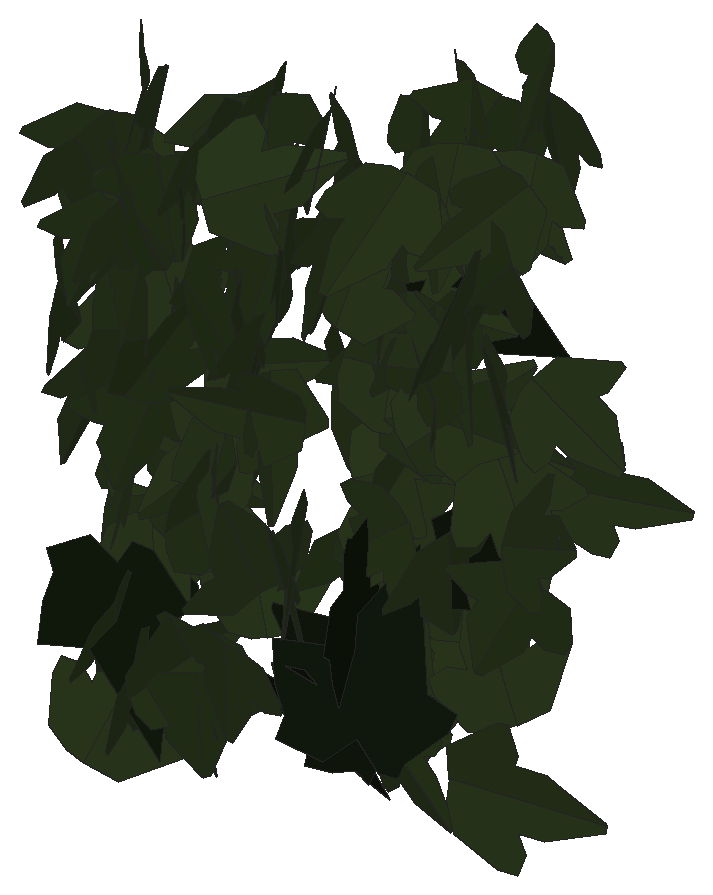
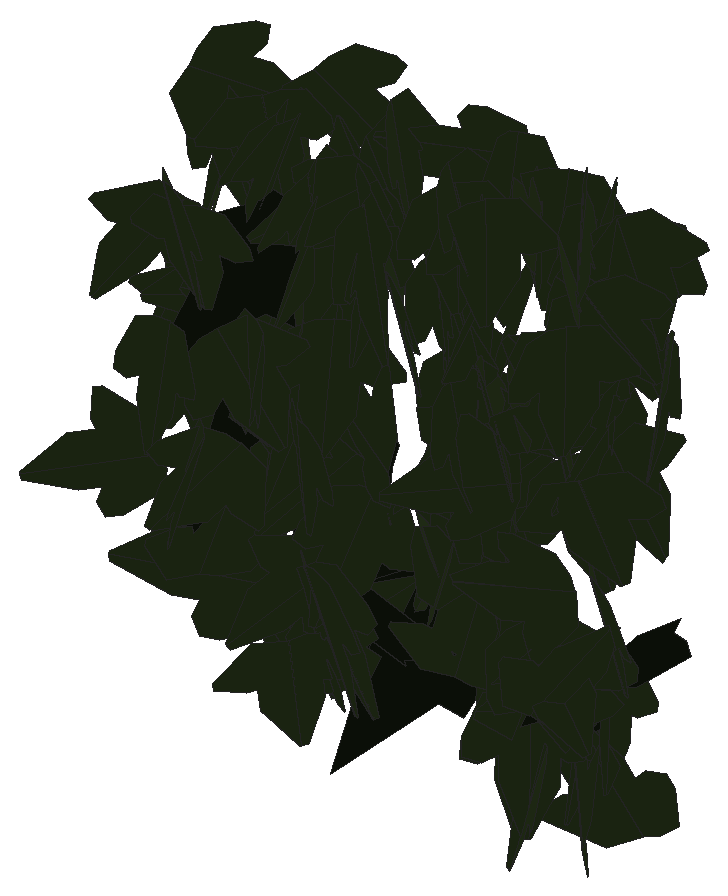
# SketchUp Ruby script. Lengths in inches.
U = 1.inch
M = Sketchup.active_model
def pt(a) = Geom::Point3d.new(a.map { |v| v * U })
def face(e, loops, mat)
  f = e.add_face(loops[0].map { |a| pt(a) })
  loops[1..].each { |l| e.add_face(l.map { |a| pt(a) }).erase! }
  f.material = f.back_material = mat if mat
  f
end
# faces: each face lists its corners as indices into pts; further lists are holes
def faces(e, pts, list, mat = nil) = list.each { |f| face(e, (f[0].is_a?(Array) ? f : [f]).map { |l| l.map { |i| pts[i] } }, mat) }
# xy, xz, yz: faces in a plane at the given z, y or x. An outline is a flat list of corners, or four numbers for a rectangle; further outlines are holes
def ring(l) = l.size == 4 ? [[l[0], l[1]], [l[2], l[1]], [l[2], l[3]], [l[0], l[3]]] : l.each_slice(2).to_a
def flat(e, list, mat, &to3) = list.each { |f| face(e, (f[0].is_a?(Array) ? f : [f]).map { |l| ring(l).map { |u, v| to3.(u, v) } }, mat) }
def xy(e, z, list, mat = nil) = flat(e, list, mat) { |x, y| [x, y, z] }
def xz(e, y, list, mat = nil) = flat(e, list, mat) { |x, z| [x, y, z] }
def yz(e, x, list, mat = nil) = flat(e, list, mat) { |y, z| [x, y, z] }
def lines(e, pts, list) = list.each { |a, b| e.add_line(pt(pts[a]), pt(pts[b])) }
# prism: a flat outline (further loops are holes) pulled along v
def prism(e, loops, v, mat = nil)
  f = face(e, loops, mat); d = Geom::Vector3d.new(v.map { |x| x * U })
  f.pushpull(f.normal.samedirection?(d) ? d.length : -d.length)
end
def box(e, o, s, mat = nil) = prism(e, [[o, [o[0] + s[0], o[1], o[2]], [o[0] + s[0], o[1] + s[1], o[2]], [o[0], o[1] + s[1], o[2]]]], [0, 0, s[2]], mat)
def at(x, y, z, deg = 0) = Geom::Transformation.translation(pt([x, y, z])) * Geom::Transformation.rotation(ORIGIN, Z_AXIS, deg.degrees)
def axes(o, x, y, z) = Geom::Transformation.new([*x, 0, *y, 0, *z, 0, *pt(o).to_a, 1])
def part(name) = M.definitions.add(name)
# library, detail: a bought-in or finely detailed component or shape, given as its bounding box
def library(name, o, s) = part(name).tap { |d| box(d.entities, o, s) }
def detail(e, o, s) = box(e.add_group.entities, o, s)
def put(e, d, t, mat = nil) = e.add_instance(d, t).tap { |i| i.material = mat if mat }
def group(e, t, mat = nil) = e.add_group.tap { |g| g.transformation = t; g.material = mat if mat }.entities
root = M.entities
M.materials.add("efeu1").color = [18, 25, 13]
M.materials.add("efeu2").color = [43, 57, 29]
c1 = part("ivyleaf_10")
p = [[0,0.5,-0.03],[-0.0625,2.02,-0.43],[-0.19,2.01,-0.46],[-0.54,1.05,-0.29],[-0.52,0.625,-0.18],[-0.83,0.76,-0.28],
  [-1.16,0.64,-0.33],[-1.15,0.33,-0.24],[-0.77,-0.39,0.02],[-0.3,-0.51,0.16],[0.04,-0.48,0.23],[-0.02,2.01,-0.4375],
  [-0.06,2.01,-0.43],[0.04,-0.49,0.23],[0.67,-0.49,0.14],[1.38,0.36,-0.2],[1.375,0.51,-0.24],[0.81,0.65,-0.19],
  [0.62,0.59,-0.15],[0.6,1.09,-0.28],[0.5,1.23,-0.31]]
faces(c1.entities,p,[[0,1,2,3,4,5,6,7,8,9,10],[11,12,0,13,14,15,16,17,18,19,20]],"efeu2")
c2 = part("ivyleaf_9")
p = [[1.54,2.16,1.25],[1.36,2.04,1.19],[-0.21,0.99,0.68],[-0.71,1.11,0.82],[-0.85,0.86,0.67],[-0.8,0.17,0.21],
  [-0.9,-0.01,0.1],[-0.67,-0.16,-0.02],[-0.08,-0.08,-0.05],[-0.03,-0.6,-0.4],[0.65,-0.88,-0.66],[0.83,-0.6,-0.49],
  [1.29,-0.42,-0.43],[1.8125,-0.07,-0.26],[1.21,0.44,0.15]]
faces(c2.entities,p,[[0,1,2,3,4,5,6,7,8,9,10,11,12,13,14]],"efeu1")
put(root,c1,axes([517.64,137.4375,171.26],[-0.41688,-0.46521,0.2029],[-0.12447,-0.16084,-0.62452],[0.49204,-0.43484,0.01392]))
put(root,c1,axes([517.58,138.02,170.76],[0.50055,0.26687,-0.30251],[-0.27279,-0.13124,-0.56713],[-0.29719,0.56995,0.01106]))
put(root,c1,axes([517.57,136.68,169.37],[0.25676,-0.43077,-0.48205],[-0.05354,0.50272,-0.47777],[0.64426,0.21346,0.15241]))
put(root,c1,axes([517.52,138.27,168.3],[0.55314,0.38276,-0.16418],[-0.12927,-0.1017,-0.67259],[-0.39592,0.56796,-0.00978]))
put(root,c1,axes([517.625,137.09,171.14],[-0.27738,-0.54194,-0.30528],[0.1181,0.2823,-0.60844],[0.6107,-0.30074,-0.021]))
put(root,c1,axes([517.77,137.28,168.16],[0.02051,-0.62852,0.23191],[0.01492,-0.23153,-0.62881],[0.66977,0.02441,0.0069]))
put(root,c1,axes([517.74,138.43,170.21],[-0.36359,-0.52843,0.00032],[0.09695,-0.06709,-0.6305],[0.51946,-0.35734,0.1179]))
put(root,c1,axes([517.9375,137.78,171.82],[0.11467,-0.29115,-0.5829],[-0.19247,0.55031,-0.31273],[0.62249,0.22379,0.01068]))
put(root,c1,axes([517.8125,137.65,166.57],[0.49001,-0.44367,0.04357],[0.03635,-0.02476,-0.661],[0.44432,0.49132,0.00603]))
put(root,c1,axes([518.02,137.22,170.3],[-0.24186,-0.56119,0.25106],[-0.10207,-0.22939,-0.61109],[0.60626,-0.2625,-0.00272]))
put(root,c1,axes([517.92,137.14,168.78],[0.08283,-0.33916,-0.69143],[0.11937,0.69267,-0.32546],[0.76083,-0.07175,0.12634]))
put(root,c1,axes([517.83,138.25,171.48],[0.29503,-0.48495,0.30679],[0.20898,-0.23047,-0.56529],[0.53443,0.35784,0.05169]))
put(root,c1,axes([517.69,138.11,163.74],[-0.17301,0.10333,0.67463],[0.5676,-0.36467,0.20141],[0.37898,0.59335,0.00631]))
put(root,c1,axes([518.25,138.12,165.25],[0.33526,0.43245,0.34069],[-0.20578,-0.27154,0.54718],[0.51062,-0.39337,-0.00318]))
put(root,c1,axes([518.2,136.93,165.01],[0.05391,-0.58364,-0.27077],[-0.01616,0.2704,-0.58607],[0.64319,0.05571,0.00797]))
put(root,c1,axes([518.49,138.06,165.82],[-0.49926,-0.31226,0.34526],[-0.2853,-0.19481,-0.58875],[0.36786,-0.5749,0.01198]))
put(root,c1,axes([518.2,137.67,170.58],[-0.05586,-0.45061,0.49221],[0.07276,-0.4951,-0.445],[0.66335,0.01636,0.09026]))
put(root,c1,axes([518.41,137.38,167.77],[-0.42657,-0.46754,0.19759],[-0.13608,-0.1433,-0.63288],[0.489,-0.44773,-0.00377]))
put(root,c1,axes([518.29,137.99,168.83],[0.29373,0.60761,0.09095],[-0.04537,-0.07908,0.67485],[0.6127,-0.29715,0.00637]))
put(root,c1,axes([518.34,137.83,168.84],[0.36132,-0.5316,-0.13386],[-0.06634,0.11675,-0.64268],[0.54417,0.36721,0.01054]))
put(root,c1,axes([518.16,137.77,165.625],[0.44886,0.5418,-0.00013],[-0.0055,0.00439,-0.70355],[-0.54178,0.44884,0.00704]))
put(root,c1,axes([517.99,136.96,163.29],[0.65454,0.19171,-0.32038],[0.30766,0.08937,0.68204],[0.21152,-0.72324,-0.00064]))
put(root,c1,axes([518.32,137.14,169.51],[0.5315,-0.32105,-0.18696],[-0.08148,0.21767,-0.60539],[0.36248,0.51968,0.13806]))
put(root,c2,axes([518.04,137.26,165.41],[0.04679,-0.74995,-0.27279],[-0.01333,0.27249,-0.7514],[0.79791,0.04853,0.00345]))
put(root,c1,axes([518.4375,136.9,170.65],[-0.14155,-0.58604,-0.38884],[0.11696,0.3715,-0.60248],[0.69351,-0.18227,0.02224]))
put(root,c1,axes([518.61,136.95,170.3],[-0.45453,0.48299,-0.05741],[-0.05818,0.02403,0.66273],[0.4829,0.45751,0.0258]))
put(root,c1,axes([518.67,136.78,164.39],[0.11905,-0.52024,-0.41216],[0.00472,0.41939,-0.528],[0.6637,0.09034,0.07768]))
put(root,c1,axes([518.27,138.12,166.72],[-0.15942,0.0089,-0.64339],[0.63789,-0.08478,-0.15923],[-0.08442,-0.65741,0.01183]))
put(root,c1,axes([518.77,137.75,163.97],[-0.47433,0.45423,0.01807],[-0.01388,0.01164,-0.65674],[-0.45437,-0.47453,0.0012]))
put(root,c1,axes([518.71,138.03,169.38],[0.22855,-0.52585,0.28258],[0.13003,-0.25147,-0.57312],[0.58264,0.26239,0.01706]))
put(root,c1,axes([518.99,137.62,164.53],[-0.68946,-0.12038,0.12223],[-0.11902,-0.02894,-0.69985],[0.12355,-0.69961,0.00792]))
put(root,c1,axes([518.92,137.02,171.28],[-0.59463,-0.30584,-0.02832],[0.02471,0.01388,-0.66867],[0.30615,-0.59514,-0.00104]))
put(root,c1,axes([518.74,136.95,168.48],[-0.01587,-0.60564,0.37816],[0.0675,0.37529,0.60387],[-0.71081,0.04916,0.0489]))
put(root,c1,axes([518.98,138.34,169.26],[0.36772,-0.53312,-0.12379],[-0.07433,0.09911,-0.64762],[0.54223,0.37512,-0.00482]))
put(root,c1,axes([518.96,138.42,171.5],[-0.40198,-0.4968,0.02458],[0.08605,-0.10059,-0.62568],[0.48991,-0.38997,0.13007]))
put(root,c1,axes([518.95,136.87,164.32],[0.02781,-0.25459,0.6538],[0.00815,0.65438,0.25447],[-0.70157,-0.00249,0.02887]))
put(root,c1,axes([518.88,137.65,170.89],[0.0621,-0.27819,-0.60931],[0.17844,-0.58294,0.28433],[-0.64561,-0.18787,0.01998]))
put(root,c1,axes([519.21,137.68,167.23],[-0.15559,-0.09227,0.6372],[0.07092,-0.654,-0.07739],[0.63992,0.05005,0.1635]))
put(root,c1,axes([519.32,137.19,164.24],[-0.50827,-0.44501,-0.02178],[0.01647,0.01426,-0.67555],[0.44523,-0.50854,0.00012]))
put(root,c1,axes([519.12,141.61,169.97],[0.52221,-0.3603,0.08583],[0.12676,0.03446,-0.6266],[0.34802,0.52809,0.09944]))
put(root,c1,axes([518.94,138.34,168.02],[0.02994,-0.04889,0.63892],[0.309,0.56144,0.02849],[-0.56136,0.30643,0.04976]))
put(root,c1,axes([519.32,138.48,168.97],[0.02159,-0.63533,0.02516],[0.02441,-0.02433,-0.63526],[0.63536,0.02252,0.02355]))
put(root,c1,axes([519.36,137.3,171.73],[-0.02289,-0.62057,-0.32602],[0.0194,0.32551,-0.62095],[0.70072,-0.02928,0.00655]))
put(root,c1,axes([519.37,138.48,171.6],[-0.40551,-0.48926,0.03021],[0.04309,-0.07463,-0.63031],[0.48829,-0.39972,0.08071]))
put(root,c1,axes([519.36,138.43,171.88],[0.11507,-0.62928,0.02192],[0.00385,-0.02158,-0.63971],[0.62965,0.11514,-0.0001]))
put(root,c1,axes([519.55,137.73,169.84],[0.04002,-0.10856,-0.66867],[-0.0739,0.66514,-0.11241],[0.67338,0.07945,0.0274]))
put(root,c1,axes([519.14,137.74,167.3],[0.0355,-0.02653,-0.64087],[0.27993,-0.57686,0.03938],[-0.57711,-0.28144,-0.02031]))
put(root,c1,axes([519.54,136.96,169.83],[-0.3289,0.54085,0.3855],[-0.192,0.33438,-0.63295],[-0.63581,-0.38075,-0.00828]))
put(root,c1,axes([519.53,136.68,166.81],[0.02424,0.02111,0.65659],[-0.22978,0.6158,-0.01132],[-0.61543,-0.22909,0.03009]))
put(root,c1,axes([519.85,137.75,169.22],[0.23119,-0.09019,0.62127],[-0.58524,0.20861,0.24807],[-0.22717,-0.62921,-0.0068]))
put(root,c1,axes([519.42,138.15,167.35],[-0.06097,-0.02228,0.65518],[0.31749,-0.57669,0.00994],[0.57355,0.31686,0.06415]))
put(root,c1,axes([519.56,137.43,167.72],[0.25378,0.61188,-0.14748],[-0.05329,-0.13756,-0.66241],[-0.62714,0.25929,-0.00339]))
put(root,c1,axes([519.72,137.94,165.18],[0.57225,0.27682,0.15029],[-0.13842,-0.05897,0.63565],[0.28294,-0.58871,0.007]))
put(root,c1,axes([519.8,137.72,169.11],[0.09402,-0.6424,0.03786],[0.00407,-0.03767,-0.64925],[0.64351,0.0941,-0.00143]))
put(root,c1,axes([519.93,138.01,170.28],[-0.14502,-0.61082,0.15015],[-0.03017,-0.14715,-0.62778],[0.62827,-0.14805,0.00451]))
put(root,c1,axes([520.03,136.91,165.01],[-0.6357,0.03884,0.16465],[-0.16466,0.00483,-0.63686],[-0.03881,-0.65666,0.00505]))
put(root,c1,axes([520.33,137.43,168.22],[-0.13923,0.09197,-0.63195],[-0.62403,-0.15699,0.11463],[-0.13566,0.62777,0.12125]))
put(root,c1,axes([519.99,137.49,165.91],[-0.30786,-0.56385,-0.32507],[-0.14344,-0.29198,0.64229],[-0.63484,0.3394,0.01251]))
put(root,c1,axes([519.91,138.03,170.32],[0.39093,-0.51019,-0.0648],[0.05112,0.11954,-0.63278],[0.51174,0.3778,0.11272]))
put(root,c1,axes([519.92,141.5625,170.86],[-0.46716,0.41506,-0.1659],[0.04195,-0.1982,-0.614],[-0.44501,-0.4544,0.11628]))
put(root,c1,axes([519.9,137.94,168.07],[-0.02344,0.68269,-0.2239],[0.01447,-0.22352,-0.68306],[-0.71832,-0.02678,-0.00645]))
put(root,c1,axes([520.42,138.91,171.07],[-0.49785,0.20256,0.52864],[-0.50472,0.16004,-0.53665],[-0.25641,-0.70831,0.02992]))
put(root,c1,axes([520.33,141.51,170.66],[-0.41762,-0.37017,0.33114],[-0.21401,-0.2563,-0.55642],[0.44819,-0.4673,0.04287]))
put(root,c1,axes([520.34,137.52,170.77],[0.00828,0.21516,-0.621],[-0.17314,0.59982,0.20552],[0.634,0.161,0.06424]))
put(root,c1,axes([520.15,142.44,169.74],[-0.31556,0.55437,-0.02515],[0.02061,-0.01721,-0.63782],[-0.55455,-0.31609,-0.00939]))
put(root,c1,axes([520.29,138.41,170.125],[0.44141,-0.46826,-0.02029],[-0.00115,0.02678,-0.64328],[0.4687,0.44107,0.01752]))
put(root,c1,axes([520.14,141.92,169.46],[-0.45097,-0.22462,-0.39564],[0.41045,0.03946,-0.49025],[0.19627,-0.59863,0.11614]))
put(root,c1,axes([519.99,136.97,171.48],[0.19355,-0.00511,-0.67426],[0.58077,0.35766,0.164],[0.34258,-0.60346,0.10291]))
put(root,c1,axes([520.58,137.99,172.07],[0.20739,-0.62861,-0.08831],[-0.01157,0.08915,-0.66172],[0.63468,0.20703,0.01679]))
put(root,c1,axes([520.375,137.47,166.28],[-0.37386,0.46001,-0.27352],[0.18004,-0.2061,-0.5927],[-0.50399,-0.41486,-0.00884]))
put(root,c1,axes([520.65,138.36,170.49],[0.06241,-0.59673,-0.24058],[0.10624,0.24795,-0.58745],[0.63457,0.01718,0.12201]))
put(root,c1,axes([520.53,137.57,166.7],[0.28508,-0.28805,0.53632],[0.38759,-0.37081,-0.40517],[0.46946,0.48105,0.00883]))
put(root,c1,axes([520.33,138.65,168.07],[-0.10454,-0.0025,0.74605],[0.71745,-0.20696,0.09984],[0.20463,0.72435,0.0311]))
put(root,c1,axes([521.01,141.96,170.71],[-0.61169,0.19732,0.08542],[-0.08791,0.00557,-0.64237],[-0.19623,-0.6176,0.0215]))
put(root,c1,axes([521.15,138.71,165.92],[0.56927,-0.28984,-0.4175],[-0.35146,0.22834,-0.63774],[0.36713,0.66801,0.03685]))
put(root,c2,axes([520.75,137.01,164.91],[0.74936,0.1265,-0.10238],[-0.10095,-0.01703,-0.75996],[-0.12764,0.75613,0.00002]))
put(root,c1,axes([521.2,138.71,165.92],[0.5832,-0.47068,-0.14626],[-0.11538,0.08991,-0.74943],[0.47918,0.5945,-0.00245]))
put(root,c1,axes([521.14,137.99,166.63],[-0.37029,-0.48383,-0.30882],[0.18133,0.25008,-0.60922],[0.54459,-0.41224,-0.00713]))
put(root,c1,axes([521.32,138.375,169.02],[-0.46453,-0.45378,-0.04907],[0.02882,0.04071,-0.64933],[0.45552,-0.46534,-0.00896]))
put(root,c1,axes([521.29,137.49,171.17],[0.10146,-0.62963,0.21567],[0.07532,-0.20589,-0.63653],[0.66127,0.12006,0.03941]))
put(root,c2,axes([521.93,137.35,164.93],[-0.53326,-0.03605,-0.56706],[-0.55591,-0.12779,0.5309],[-0.11755,0.76784,0.06173]))
put(root,c1,axes([521.58,140.96,171.99],[0.45997,-0.43119,-0.08942],[-0.05346,0.07367,-0.63024],[0.43711,0.46275,0.01702]))
put(root,c1,axes([521.69,138.05,164.73],[0.02404,0.2892,0.67807],[-0.07076,-0.6744,0.29014],[0.73377,-0.07451,0.00577]))
put(root,c1,axes([521.32,137.98,170.93],[-0.1875,-0.20395,-0.57631],[0.48447,0.31807,-0.27018],[0.37285,-0.51586,0.06125]))
put(root,c1,axes([522.01,137.49,167.27],[0.39783,-0.14512,-0.48941],[-0.43301,0.23265,-0.42098],[0.27033,0.58623,0.04592]))
put(root,c1,axes([521.53,137.32,170.33],[0.66433,-0.11572,-0.11217],[0.1173,0.02094,0.67313],[-0.11051,-0.6734,0.0402]))
put(root,c1,axes([521.65,138.42,171.1],[0.00527,0.59662,-0.23108],[-0.0124,-0.23095,-0.59656],[-0.63969,0.0094,0.00966]))
put(root,c2,axes([521.93,136.76,166.6875],[0.12356,-0.06211,-0.76596],[-0.62775,0.43933,-0.13689],[0.44326,0.63949,0.01965]))
put(root,c1,axes([521.69,138.65,164.85],[0.44545,0.50513,-0.06677],[-0.04805,-0.04665,-0.67347],[-0.50726,0.448,0.00516]))
put(root,c1,axes([521.77,138.15,168.03],[-0.10534,-0.50237,-0.46448],[0.10769,0.45192,-0.51321],[0.67567,-0.15035,0.00938]))
put(root,c1,axes([521.78,137.95,170.375],[0.12684,-0.4773,-0.50678],[0.09194,0.52209,-0.46871],[0.69006,0.01817,0.1556]))
put(root,c1,axes([521.57,138.34,165.85],[0.24648,0.26016,0.53209],[0.2024,0.50463,-0.34049],[-0.55663,0.29869,0.1118]))
put(root,c1,axes([521.6,137.9,167.1],[0.34053,0.33834,0.47524],[0.30306,0.3676,-0.47886],[-0.49848,0.45462,0.03352]))
put(root,c1,axes([521.8125,137.95,164.28],[0.63523,-0.26037,-0.02043],[0.03129,0.02252,0.68574],[-0.25929,-0.63516,0.03269]))
put(root,c1,axes([521.53,137.95,167.72],[0.18462,-0.03693,-0.66129],[0.58628,0.32849,0.14533],[0.30813,-0.6029,0.11969]))
put(root,c1,axes([522.23,138.12,169.91],[-0.47199,-0.30961,0.2979],[-0.23487,-0.18464,-0.56402],[0.35978,-0.52671,0.02261]))
put(root,c1,axes([522.11,137.39,171.89],[0.41655,0.3968,-0.3783],[-0.28964,-0.24411,-0.57497],[-0.46548,0.50699,0.01924]))
put(root,c1,axes([522.04,138.39,171.58],[-0.11656,0.61723,0.13735],[-0.01088,0.13768,-0.62797],[-0.63223,-0.11616,-0.01452]))
put(root,c1,axes([521.79,137.44,169.45],[0.15828,0.14682,0.65035],[0.28083,0.59156,-0.2019],[-0.60469,0.31316,0.07647]))
put(root,c2,axes([522.1,136.79,164.84],[-0.64803,0.06814,0.51258],[0.50175,-0.11585,0.64973],[0.12503,0.81808,0.04932]))
put(root,c1,axes([522.19,138,169.81],[-0.20194,-0.57345,-0.30825],[0.13013,0.28067,-0.6074],[0.63791,-0.23879,0.02632]))
put(root,c1,axes([522.52,137.57,169.32],[0.11206,0.00148,-0.71032],[-0.34806,0.62698,-0.0536],[0.61921,0.35216,0.09842]))
put(root,c1,axes([521.78,138.125,170.07],[-0.16223,-0.13455,-0.64567],[0.61692,0.20418,-0.19755],[0.23324,-0.63366,0.07344]))
put(root,c2,axes([522.02,138.39,170.27],[0.03164,-0.12649,-0.76017],[-0.09585,0.75426,-0.12949],[0.76464,0.09978,0.01523]))
put(root,c1,axes([522.16,138.37,171.7],[0.0787,0.61377,-0.17832],[-0.0226,-0.17689,-0.61879],[-0.63875,0.08188,-0.00008]))
put(root,c1,axes([522.24,138.42,171.875],[0.47127,0.42567,-0.08953],[-0.11605,-0.00418,-0.63073],[-0.41921,0.47968,0.07396]))
put(root,c1,axes([522.81,137.42,169.77],[-0.18012,0.04238,0.65889],[-0.65548,-0.09347,-0.17317],[0.07926,-0.67664,0.06519]))
put(root,c1,axes([522.22,139.91,171.08],[0.63318,0.07836,-0.00643],[-0.006,-0.00382,-0.638],[-0.0784,0.6332,-0.00305]))
put(root,c1,axes([522.27,137.25,164.57],[-0.39184,0.14245,-0.49831],[0.44953,-0.21748,-0.41566],[-0.25793,-0.59544,0.0326]))
put(root,c1,axes([522.13,137.73,168.77],[-0.01117,-0.0111,-0.6802],[0.64845,0.20552,-0.014],[0.2057,-0.6485,0.0072]))
put(root,c2,axes([522.93,138.36,166.66],[-0.20088,-0.46113,0.58993],[0.23388,0.54159,0.50298],[-0.71131,0.3083,-0.00121]))
put(root,c1,axes([522.49,137.68,168.74],[0.18875,0.21563,-0.65889],[0.48227,0.44973,0.28534],[0.49804,-0.51721,-0.02659]))
put(root,c1,axes([522.98,137.38,167.38],[-0.08685,-0.7106,-0.1792],[0.03661,0.17602,-0.71574],[0.73193,-0.09312,0.01453]))
put(root,c1,axes([523.34,138.1,171.9375],[0.1876,0.28807,-0.55174],[-0.39372,-0.39139,-0.33822],[-0.48206,0.43177,0.06153]))
put(root,c1,axes([522.8,137.84,170.02],[0.38785,-0.23679,0.45324],[0.41671,-0.18337,-0.45238],[0.29639,0.56765,0.04293]))
put(root,c1,axes([523.58,137.8,171.21],[-0.40996,0.13846,0.48236],[-0.4867,0.04215,-0.42575],[-0.12235,-0.63163,0.07733]))
put(root,c1,axes([523.1,137.03,170.18],[0.20953,-0.71333,0.09203],[0.02392,0.10271,0.74168],[-0.71884,-0.20451,0.05151]))
put(root,c1,axes([523.47,137.91,165.31],[0.31107,0.64651,0.10986],[-0.05549,-0.09521,0.7174],[0.65342,-0.31586,0.00862]))
put(root,c1,axes([523.02,137.67,168.86],[0.10266,0.0143,0.67953],[0.56981,0.37283,-0.09393],[-0.37052,0.57732,0.04383]))
put(root,c1,axes([523.37,139.49,167.34],[0.12018,0.00111,0.64955],[0.42275,0.50138,-0.07907],[-0.49314,0.43009,0.09051]))
put(root,c1,axes([524.27,137.22,167.22],[-0.56294,-0.21896,0.34265],[-0.30725,-0.15427,-0.60337],[0.26636,-0.64071,0.02818]))
put(root,c1,axes([523.95,137.07,170.3125],[-0.40702,0.51378,-0.15067],[0.08574,-0.12427,-0.65539],[-0.52851,-0.41584,0.00971]))
put(root,c1,axes([523.8,137.49,168.46],[0.53444,0.34047,0.27122],[0.22387,0.15334,-0.63363],[-0.37332,0.57938,0.00831]))
put(root,c1,axes([523.77,137.01,164.48],[0.01736,-0.04195,0.81892],[0.73597,0.36199,0.00294],[-0.36158,0.73478,0.0453]))
put(root,c1,axes([524.17,137.91,169.62],[0.24307,0.43634,0.43011],[0.18859,0.38697,-0.49915],[-0.58294,0.30713,0.01786]))
put(root,c1,axes([524.57,136.84,168.1875],[-0.09078,0.27104,0.60208],[-0.21042,0.56418,-0.28571],[-0.62585,-0.229,0.00873]))
